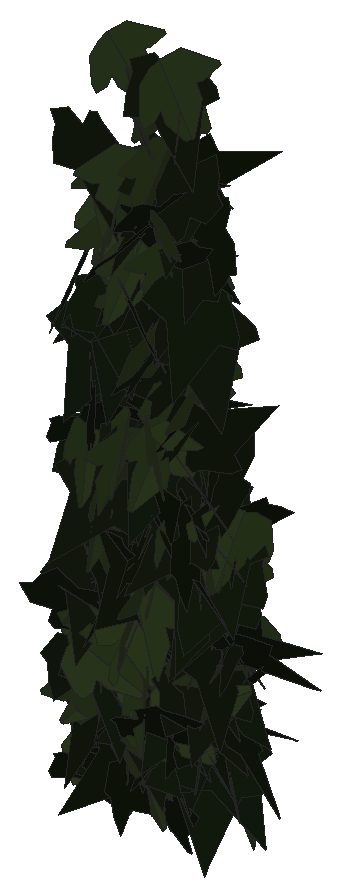
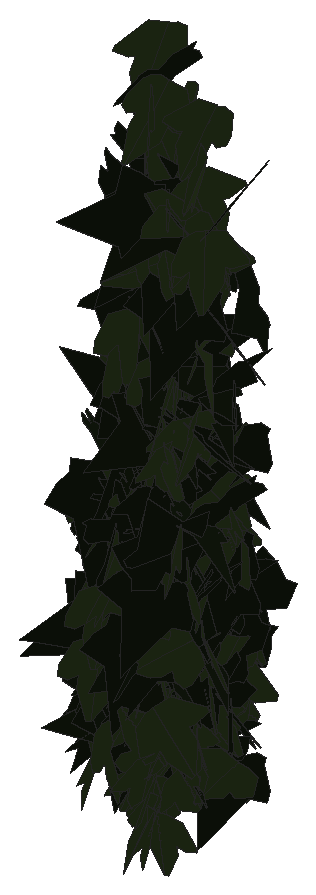
# SketchUp Ruby script. Lengths in inches.
U = 1.inch
M = Sketchup.active_model
def pt(a) = Geom::Point3d.new(a.map { |v| v * U })
def face(e, loops, mat)
  f = e.add_face(loops[0].map { |a| pt(a) })
  loops[1..].each { |l| e.add_face(l.map { |a| pt(a) }).erase! }
  f.material = f.back_material = mat if mat
  f
end
# faces: each face lists its corners as indices into pts; further lists are holes
def faces(e, pts, list, mat = nil) = list.each { |f| face(e, (f[0].is_a?(Array) ? f : [f]).map { |l| l.map { |i| pts[i] } }, mat) }
# xy, xz, yz: faces in a plane at the given z, y or x. An outline is a flat list of corners, or four numbers for a rectangle; further outlines are holes
def ring(l) = l.size == 4 ? [[l[0], l[1]], [l[2], l[1]], [l[2], l[3]], [l[0], l[3]]] : l.each_slice(2).to_a
def flat(e, list, mat, &to3) = list.each { |f| face(e, (f[0].is_a?(Array) ? f : [f]).map { |l| ring(l).map { |u, v| to3.(u, v) } }, mat) }
def xy(e, z, list, mat = nil) = flat(e, list, mat) { |x, y| [x, y, z] }
def xz(e, y, list, mat = nil) = flat(e, list, mat) { |x, z| [x, y, z] }
def yz(e, x, list, mat = nil) = flat(e, list, mat) { |y, z| [x, y, z] }
def lines(e, pts, list) = list.each { |a, b| e.add_line(pt(pts[a]), pt(pts[b])) }
# prism: a flat outline (further loops are holes) pulled along v
def prism(e, loops, v, mat = nil)
  f = face(e, loops, mat); d = Geom::Vector3d.new(v.map { |x| x * U })
  f.pushpull(f.normal.samedirection?(d) ? d.length : -d.length)
end
def box(e, o, s, mat = nil) = prism(e, [[o, [o[0] + s[0], o[1], o[2]], [o[0] + s[0], o[1] + s[1], o[2]], [o[0], o[1] + s[1], o[2]]]], [0, 0, s[2]], mat)
def at(x, y, z, deg = 0) = Geom::Transformation.translation(pt([x, y, z])) * Geom::Transformation.rotation(ORIGIN, Z_AXIS, deg.degrees)
def axes(o, x, y, z) = Geom::Transformation.new([*x, 0, *y, 0, *z, 0, *pt(o).to_a, 1])
def part(name) = M.definitions.add(name)
# library, detail: a bought-in or finely detailed component or shape, given as its bounding box
def library(name, o, s) = part(name).tap { |d| box(d.entities, o, s) }
def detail(e, o, s) = box(e.add_group.entities, o, s)
def put(e, d, t, mat = nil) = e.add_instance(d, t).tap { |i| i.material = mat if mat }
def group(e, t, mat = nil) = e.add_group.tap { |g| g.transformation = t; g.material = mat if mat }.entities
root = M.entities
M.materials.add("efeu1").color = [18, 25, 13]
M.materials.add("efeu2").color = [43, 57, 29]
c1 = part("ivyleaf_10")
p = [[0,0.5,-0.03],[-0.0625,2.02,-0.43],[-0.19,2.01,-0.46],[-0.54,1.05,-0.29],[-0.52,0.625,-0.18],[-0.83,0.76,-0.28],
  [-1.16,0.64,-0.33],[-1.15,0.33,-0.24],[-0.77,-0.39,0.02],[-0.3,-0.51,0.16],[0.04,-0.48,0.23],[-0.02,2.01,-0.4375],
  [-0.06,2.01,-0.43],[0.04,-0.49,0.23],[0.67,-0.49,0.14],[1.38,0.36,-0.2],[1.375,0.51,-0.24],[0.81,0.65,-0.19],
  [0.62,0.59,-0.15],[0.6,1.09,-0.28],[0.5,1.23,-0.31]]
faces(c1.entities,p,[[0,1,2,3,4,5,6,7,8,9,10],[11,12,0,13,14,15,16,17,18,19,20]],"efeu2")
c2 = part("ivyleaf_9")
p = [[1.54,2.16,1.25],[1.36,2.04,1.19],[-0.21,0.99,0.68],[-0.71,1.11,0.82],[-0.85,0.86,0.67],[-0.8,0.17,0.21],
  [-0.9,-0.01,0.1],[-0.67,-0.16,-0.02],[-0.08,-0.08,-0.05],[-0.03,-0.6,-0.4],[0.65,-0.88,-0.66],[0.83,-0.6,-0.49],
  [1.29,-0.42,-0.43],[1.8125,-0.07,-0.26],[1.21,0.44,0.15]]
faces(c2.entities,p,[[0,1,2,3,4,5,6,7,8,9,10,11,12,13,14]],"efeu1")
put(root,c1,axes([7.61,224.5,225.21],[0.35894,-0.31903,0.13922],[0.09481,-0.10282,-0.48004],[0.33492,0.37101,-0.01332]))
put(root,c1,axes([7.58,224.07,225.04],[0.18757,0.37221,0.14899],[0.06063,0.13188,-0.42714],[-0.42644,0.18247,0.00481]))
put(root,c1,axes([7.75,224.44,231.33],[-0.22715,-0.3782,-0.04595],[0.02733,0.03648,-0.45004],[0.41032,-0.2118,0.00454]))
put(root,c2,axes([7.99,224.41,227.15],[-0.21542,0.37118,0.11234],[-0.11464,0.06429,-0.4336],[-0.40145,-0.21753,0.06354]))
put(root,c1,axes([7.73,224.59,228.66],[0.07574,-0.26071,-0.35473],[0.02197,0.34723,-0.27168],[0.46313,0.02617,0.0709]))
put(root,c2,axes([7.83,223.22,229.9],[0.04008,0.18203,0.40907],[0.01412,0.39413,-0.19097],[-0.46787,0.02749,0.02928]))
put(root,c2,axes([7.56,224.16,223.65],[-0.02545,0.09105,0.4417],[0.06137,-0.42104,0.09715],[0.46508,0.06054,0.01135]))
put(root,c2,axes([7.57,224.38,227.42],[0.00542,-0.49083,-0.09518],[0.00382,0.09522,-0.49083],[0.49996,0.0046,0.00479]))
put(root,c1,axes([7.64,225.54,222.95],[0.46659,-0.00564,0.05248],[0.05452,0.0009,-0.44934],[0.00593,0.43496,0.00161]))
put(root,c1,axes([7.77,224.16,227.36],[0.17335,0.3156,-0.26281],[-0.12938,-0.22256,-0.3682],[-0.41704,0.20023,0.00498]))
put(root,c1,axes([7.8,225.07,227.125],[-0.37043,0.26625,0.02742],[-0.04567,-0.01161,-0.4501],[-0.28532,-0.34381,0.03644]))
put(root,c2,axes([7.73,223.81,223.13],[0.3453,0.28887,-0.06203],[-0.05186,-0.03581,-0.44809],[-0.31431,0.32326,0.00578]))
put(root,c1,axes([7.9,225.1875,224.25],[-0.17476,-0.34873,0.21168],[-0.08556,-0.18759,-0.39977],[0.42761,-0.18006,0.00652]))
put(root,c2,axes([8.05,224.07,225.14],[-0.1459,0.38314,0.16172],[-0.08247,0.13766,-0.42174],[-0.43889,-0.15324,0.02548]))
put(root,c2,axes([7.58,223.94,231.97],[0.19819,-0.45872,-0.01728],[-0.00253,0.01773,-0.49968],[0.45904,0.19815,0.0047]))
put(root,c1,axes([7.56,224.15,223.18],[0.3046,0.18868,0.28306],[0.23736,0.1608,-0.35278],[-0.26757,0.35745,0.00928]))
put(root,c1,axes([7.86,224.03,225.55],[-0.02783,-0.49665,-0.05061],[0.00726,0.05028,-0.49741],[0.49917,-0.02843,0.00442]))
put(root,c1,axes([7.76,224.79,228.71],[0.14203,0.41463,-0.00394],[-0.01303,-0.00014,-0.45223],[-0.44763,0.13156,0.01192]))
put(root,c1,axes([8.05,223.99,229.33],[-0.03318,0.19852,0.40127],[-0.34968,0.24702,-0.15899],[-0.31199,-0.29798,0.13553]))
put(root,c2,axes([7.84,224,226],[0.30337,0.30705,-0.13173],[-0.08637,-0.09848,-0.43273],[-0.34817,0.29197,-0.00743]))
put(root,c2,axes([7.82,224.1,224.2],[-0.40754,-0.06704,-0.28181],[0.28924,-0.0676,-0.40221],[0.01583,-0.49085,0.09388]))
put(root,c2,axes([7.74,223.61,224.93],[0.07038,-0.23683,-0.37337],[-0.11954,0.34165,-0.25528],[0.44885,0.12812,-0.00944]))
put(root,c2,axes([7.45,224,224.97],[0.22302,-0.1763,0.35345],[0.31425,-0.17869,-0.28028],[0.26874,0.35526,0.03443]))
put(root,c1,axes([7.85,223.74,226.28],[-0.43437,0.16544,-0.01004],[0.00865,-0.00591,-0.45228],[-0.17877,-0.40227,0.00252]))
put(root,c2,axes([7.78,224.18,229.08],[-0.14899,-0.43209,0.20273],[-0.02194,-0.20595,-0.45509],[0.47678,-0.1445,0.0424]))
put(root,c1,axes([8.01,224.08,224.32],[0.21632,0.21762,-0.33174],[-0.28496,-0.18523,-0.30374],[-0.30449,0.32796,0.04858]))
put(root,c1,axes([7.93,223.73,224.32],[-0.42115,-0.26938,-0.0083],[0.00407,0.00904,-0.4999],[0.26947,-0.42113,-0.00543]))
put(root,c2,axes([7.88,225.1,226.84],[-0.24224,-0.1765,0.3414],[0.27838,0.20327,0.29683],[-0.29075,0.34169,-0.00023]))
put(root,c1,axes([7.61,224.95,226.38],[0.22392,-0.13062,0.37379],[0.35999,-0.13865,-0.25238],[0.20242,0.39108,0.03536]))
put(root,c1,axes([7.82,224.49,232.58],[-0.27933,0.33329,-0.11032],[0.06892,-0.08475,-0.43874],[-0.3714,-0.26639,0.00156]))
put(root,c2,axes([8.1875,224.59,228.57],[-0.44129,0.12207,0.08927],[-0.10108,-0.01474,-0.44154],[-0.12552,-0.41726,0.04172]))
put(root,c1,axes([8.01,224.25,224.0625],[0.38812,0.09295,-0.23588],[-0.23564,-0.06213,-0.38601],[-0.12064,0.42039,-0.0049]))
put(root,c2,axes([7.92,223.91,225.8125],[0.12768,0.37309,0.19747],[0.06273,0.18078,-0.40703],[-0.44775,0.13171,-0.00071]))
put(root,c1,axes([7.85,225.43,222.92],[-0.16645,0.40487,-0.04095],[0.00816,-0.03925,-0.45049],[-0.43925,-0.15416,0.00715]))
put(root,c2,axes([7.85,223.58,228.125],[0.30554,0.33028,0.01032],[0.00708,0.00745,-0.45228],[-0.3568,0.28299,-0.00014]))
put(root,c1,axes([7.93,225.4375,223],[-0.13999,0.33376,0.25692],[-0.09144,0.23211,-0.37235],[-0.43904,-0.15476,-0.00437]))
put(root,c1,axes([8.04,224.125,224.58],[0.23939,-0.2391,-0.29948],[-0.17561,0.23993,-0.33735],[0.3641,0.27293,0.0342]))
put(root,c1,axes([7.9,224.76,223.25],[0.04747,0.37222,-0.22961],[-0.08439,-0.21144,-0.38692],[-0.45971,0.07725,0.04732]))
put(root,c1,axes([7.89,223.7,227.875],[0.07852,0.39784,-0.16661],[-0.02727,-0.15823,-0.42059],[-0.46239,0.07689,-0.00349]))
put(root,c1,axes([7.8,225.01,227.94],[0.22296,-0.35751,-0.14257],[0.07711,-0.11706,0.42934],[-0.40627,-0.21842,0.00325]))
put(root,c2,axes([7.5625,223.43,225.39],[0.14224,-0.0871,0.42154],[0.44001,-0.05156,-0.1492],[0.08291,0.42306,0.0686]))
put(root,c2,axes([8.21,224.7,228.48],[-0.44022,-0.05088,0.14886],[-0.14545,-0.06858,-0.42422],[0.0759,-0.42654,0.05045]))
put(root,c2,axes([7.93,223.71,226.42],[0.39807,0.13767,-0.19294],[-0.19397,-0.04895,-0.40888],[-0.15693,0.40973,0.01597]))
put(root,c1,axes([7.86,225.42,223.04],[-0.22501,0.34827,-0.16287],[0.08093,-0.13764,-0.42202],[-0.40439,-0.22133,0.00617]))
put(root,c2,axes([7.85,225.18,226.67],[0.30659,0.24189,0.23285],[-0.20101,-0.12623,0.38725],[0.29379,-0.3388,0.02196]))
put(root,c2,axes([7.73,224.65,228.18],[0.15735,-0.4086,0.03366],[0.01971,-0.02785,-0.45107],[0.44223,0.14662,0.00813]))
put(root,c2,axes([7.89,223.875,225.9],[-0.13806,-0.41381,0.04223],[-0.01431,-0.0384,-0.45042],[0.44883,-0.12851,-0.00137]))
put(root,c2,axes([7.65,224.32,224.29],[-0.01325,-0.0949,0.44132],[0.46657,-0.05094,0.00114],[0.05341,0.42146,0.09951]))
put(root,c1,axes([8.05,223.89,226.66],[-0.33491,-0.30505,-0.00273],[-0.0001,0.00383,-0.45238],[0.32946,-0.31009,-0.00291]))
put(root,c1,axes([7.96,225.38,223.27],[-0.21708,0.38487,-0.02748],[-0.00924,-0.03423,-0.45091],[-0.41654,-0.19982,0.02433]))
put(root,c1,axes([7.92,224.16,233.16],[0.17949,0.3432,0.2177],[-0.00285,0.22743,-0.38563],[-0.43415,0.1404,0.09254]))
put(root,c1,axes([8.17,223.5,225.22],[0.36409,-0.04043,-0.2828],[-0.28527,0.07166,-0.35164],[0.08232,0.42715,0.03222]))
put(root,c2,axes([8.21,223.84,229.11],[-0.19624,0.45873,0.03253],[-0.00754,0.03216,-0.49891],[-0.45982,-0.1963,-0.0057]))
put(root,c1,axes([7.69,225.04,225.4375],[0.28719,0.00254,0.35802],[0.31618,0.22719,-0.23694],[-0.19561,0.37095,0.14266]))
put(root,c1,axes([7.94,224.11,224.57],[0.1516,0.40842,-0.05418],[-0.02607,-0.04678,-0.44907],[-0.4439,0.14223,0.00787]))
put(root,c2,axes([8.24,223.94,230.13],[-0.46658,0.17785,-0.02602],[0.02806,0.00058,-0.49921],[-0.17754,-0.4673,-0.01052]))
put(root,c1,axes([7.93,223.85,227.09],[0.38214,-0.23782,0.08986],[0.07415,-0.05274,-0.44335],[0.26303,0.36039,-0.00558]))
put(root,c1,axes([7.96,224.91,228.34],[0.06858,0.42066,-0.09441],[-0.01439,-0.0898,-0.44244],[-0.46454,0.06488,-0.00023]))
put(root,c2,axes([7.97,225.16,226.3],[0.36574,0.2637,-0.07356],[-0.05036,-0.05517,-0.44612],[-0.29053,0.34153,-0.01526]))
put(root,c1,axes([8.12,224.53,223.6875],[-0.2118,-0.43639,0.12128],[-0.03301,-0.11865,-0.48459],[0.45172,-0.21328,0.02145]))
put(root,c1,axes([8,225.35,223.64],[0.03854,0.43344,0.00927],[0.00167,0.00882,-0.4523],[-0.46821,0.03571,-0.00085]))
put(root,c2,axes([8.22,223.27,228.19],[0.04121,-0.07593,0.44368],[-0.05238,0.42483,0.08315],[-0.46505,-0.05458,0.02996]))
put(root,c1,axes([8.01,225.23,223.76],[-0.0485,-0.38273,0.20987],[0.01715,0.20129,0.40071],[-0.46697,0.04715,-0.00709]))
put(root,c2,axes([7.73,224.21,225.26],[0.31805,-0.34067,0.18108],[0.15967,-0.09741,-0.4637],[0.35121,0.35279,0.04683]))
put(root,c2,axes([8.03,223.9,225.5625],[0.19457,0.27668,0.29455],[0.12601,0.26025,-0.34159],[-0.40863,0.212,0.03492]))
put(root,c1,axes([8.18,223.94,230.83],[-0.22175,-0.44636,0.03986],[-0.004,-0.0425,-0.49817],[0.44812,-0.22126,0.01528]))
put(root,c1,axes([8.07,223.77,226.95],[-0.03273,0.33799,-0.28304],[-0.0189,-0.27355,-0.35128],[-0.46828,-0.01259,0.03396]))
put(root,c2,axes([8.32,224.58,228.92],[-0.19055,0.39684,-0.02578],[0.00811,-0.02379,-0.45166],[-0.42935,-0.17657,0.00291]))
put(root,c2,axes([8.16,224.49,228.77],[-0.40195,-0.20988,-0.0849],[0.11545,-0.02585,-0.4377],[0.21406,-0.38014,0.07664]))
put(root,c1,axes([8.11,223.79,231.11],[0.32841,-0.30981,0.02892],[0.02321,-0.01787,-0.45147],[0.33514,0.30483,0.00293]))
put(root,c2,axes([7.99,224.07,224.72],[-0.03115,-0.49476,-0.06516],[0.00966,0.06468,-0.4957],[0.49894,-0.03214,0.00553]))
put(root,c1,axes([8.14,224.67,228.99],[0.1108,-0.27768,-0.33149],[0.03153,0.33186,-0.29091],[0.45546,0.04458,0.10078]))
put(root,c2,axes([8.12,224.04,223.09],[-0.3553,-0.06116,0.28907],[0.30072,0.01872,0.34703],[-0.06359,0.43027,0.02599]))
put(root,c2,axes([8.29,223.64,227.35],[-0.45345,-0.10979,-0.031],[0.03049,0.00987,-0.45133],[0.11902,-0.4208,-0.0025]))
put(root,c2,axes([8.03,223.97,225.94],[0.24739,-0.28343,-0.24704],[-0.16121,0.18478,-0.379],[0.36541,0.27341,0.00005]))
put(root,c1,axes([8.11,224.31,223.5625],[0.02926,-0.34085,0.27966],[0.11039,-0.25685,-0.3493],[0.45571,0.0841,0.06666]))
put(root,c2,axes([8.06,224.18,229.4375],[-0.09459,-0.49001,0.03076],[-0.01006,-0.02939,-0.49903],[0.49087,-0.09502,-0.0043]))
put(root,c2,axes([7.98,224.51,225.68],[0.09626,-0.49064,0.00219],[0.00039,-0.00215,-0.5],[0.49065,0.09627,-0.00003]))
put(root,c1,axes([8.2,224.625,228.96],[-0.33818,0.30184,-0.00856],[-0.04218,-0.05224,-0.44729],[-0.32337,-0.30885,0.06729]))
put(root,c2,axes([8.23,224.44,224.59],[-0.35091,0.07466,-0.2906],[0.25343,-0.17763,-0.33314],[-0.18261,-0.39,0.0961]))
put(root,c1,axes([8.24,224.2,224.51],[0.05162,-0.41708,0.11852],[0.03448,-0.11094,-0.43618],[0.46568,0.05445,0.01916]))
put(root,c1,axes([8.28,224.91,225.8],[-0.42284,0.18372,0.04866],[-0.05446,0.00257,-0.44934],[-0.19737,-0.39429,0.01974]))
put(root,c1,axes([8.27,224.26,231.46],[-0.43676,-0.15527,-0.0412],[0.03889,0.01674,-0.45051],[0.16863,-0.406,-0.00281]))
put(root,c2,axes([8.41,224.4,224.35],[-0.06273,0.42947,-0.03898],[-0.00471,-0.03841,-0.45061],[-0.46557,-0.05748,0.00982]))
put(root,c1,axes([8.18,223.88,231.0625],[0.45737,0.09911,0.00776],[0.00729,0.00389,-0.45233],[-0.1071,0.42354,0.00234]))
put(root,c1,axes([8.4,224.16,223.85],[-0.42839,-0.14086,0.11413],[-0.10976,-0.04171,-0.43774],[0.15857,-0.40944,0.00533]))
put(root,c2,axes([8.13,224.4375,226.36],[-0.04349,-0.49765,-0.02135],[0.00335,0.02113,-0.49954],[0.49809,-0.04359,0.00149]))
put(root,c2,axes([8.13,223.95,229.83],[-0.16099,-0.36088,-0.19943],[0.12995,0.15632,-0.40321],[0.42179,-0.1859,0.0481]))
put(root,c1,axes([8.03,224.2,223.5625],[0.11829,-0.10108,0.42502],[0.34507,-0.255,-0.15466],[0.29605,0.33762,0.01044]))
put(root,c1,axes([8.34,223.92,231.74],[-0.20476,-0.41564,0.18793],[0.00294,-0.2072,-0.45504],[0.45614,-0.18524,0.08729]))
put(root,c1,axes([8.29,224.03,229.15],[-0.25571,0.36272,0.04159],[-0.0315,0.0287,-0.45039],[-0.39285,-0.2384,0.00905]))
put(root,c2,axes([8.28,224.11,230.23],[0.37524,0.31312,-0.10559],[-0.11729,-0.02316,-0.4855],[-0.30892,0.38913,0.05607]))
put(root,c1,axes([8.36,224.25,230.9],[-0.06658,-0.3968,0.17395],[-0.01242,-0.16738,-0.4174],[0.46489,-0.0613,0.01376]))
put(root,c2,axes([8.51,224.25,227.93],[-0.49837,0.01119,-0.03877],[0.03888,0.00457,-0.49847],[-0.0108,-0.49985,-0.00542]))
put(root,c2,axes([7.97,223.86,222.93],[0.34235,0.04231,0.30667],[0.31579,0.03815,-0.33259],[-0.06153,0.43125,-0.00067]))
put(root,c2,axes([8.38,224.74,227.11],[-0.40489,-0.16209,-0.15567],[0.14835,0.05948,-0.42477],[0.18647,-0.39927,-0.00008]))
put(root,c2,axes([8.33,225.11,225.3],[0.34371,0.27644,-0.11164],[-0.0781,-0.08036,-0.43821],[-0.3106,0.32611,-0.01335]))
put(root,c1,axes([8.42,224.42,222.97],[-0.4695,-0.01324,0.00854],[-0.0088,-0.00222,-0.45231],[0.01434,-0.43479,0.00205]))
put(root,c2,axes([8.23,224.84,227.56],[-0.05882,-0.38552,-0.20176],[0.03162,0.19178,-0.40492],[0.46503,-0.06181,0.00201]))
put(root,c2,axes([8.4,223.85,223.45],[-0.02052,-0.09245,-0.44162],[0.17712,-0.39514,0.08183],[-0.43465,-0.15665,0.05419]))
put(root,c2,axes([8.49,223.52,230.75],[0.10655,0.45238,0.18439],[-0.02433,0.1934,-0.46044],[-0.48791,0.08915,0.06322]))
put(root,c1,axes([8.35,225.0625,225.64],[-0.14164,0.41358,-0.03248],[0.002,-0.03217,-0.45116],[-0.44793,-0.13092,0.00826]))
put(root,c1,axes([8.33,223.89,229.78],[-0.38255,-0.19027,-0.17263],[0.17746,0.04342,-0.41644],[0.20705,-0.38876,0.03798]))
put(root,c1,axes([8.24,224.25,223.1],[-0.30777,0.11338,-0.32082],[0.24081,-0.23326,-0.30338],[-0.26076,-0.34923,0.09848]))
put(root,c1,axes([8.49,223.76,227.9],[-0.05191,-0.45652,0.19721],[-0.01809,-0.19642,-0.45945],[0.49697,-0.05484,0.00388]))
put(root,c1,axes([8.2,223.27,225.06],[0.21413,0.19013,0.35078],[0.2136,0.27604,-0.28274],[-0.35949,0.27727,0.04094]))
put(root,c2,axes([8.48,223.57,223.46],[0.19308,-0.1422,-0.43875],[-0.33484,0.28388,-0.23936],[0.31718,0.38625,0.0144]))
put(root,c1,axes([8.48,224.52,224.96],[0.19428,-0.45763,-0.05317],[-0.0131,0.05219,-0.4971],[0.46053,0.19455,0.00829]))
put(root,c2,axes([8.74,224.06,223.61],[-0.26681,0.40998,0.10357],[-0.06647,0.08028,-0.48902],[-0.4176,-0.27472,0.01167]))
put(root,c1,axes([8.5,223.84,230.52],[0.19886,0.33603,-0.21416],[-0.14134,-0.16226,-0.39707],[-0.40148,0.22356,0.03371]))
put(root,c1,axes([8.375,225.04,223.875],[-0.3747,0.20373,-0.172],[0.13956,-0.10596,-0.41768],[-0.24665,-0.36945,0.02495]))
put(root,c1,axes([8.52,224.31,227.79],[0.02447,-0.4637,-0.18544],[0.01344,0.18621,-0.46384],[0.49922,0.01772,0.02158]))
put(root,c2,axes([8.14,224.25,224.91],[0.40084,-0.16238,0.1648],[0.15737,-0.06228,-0.42131],[0.18782,0.39872,0.00131]))
put(root,c1,axes([8.54,224.66,223.29],[-0.05366,-0.48467,0.11052],[0.00168,-0.11134,-0.48744],[0.49711,-0.05194,0.01357]))
put(root,c1,axes([8.3,224.07,225.63],[-0.05451,-0.13591,-0.42653],[0.31958,0.29001,-0.13782],[0.34002,-0.29436,0.06116]))
put(root,c2,axes([8.71,224.59,223.82],[-0.14377,0.3668,-0.30788],[-0.01127,-0.32395,-0.38069],[-0.47875,-0.10253,0.10141]))
put(root,c1,axes([8.71,224.37,231.56],[-0.37469,-0.1029,0.25105],[-0.1938,-0.19895,-0.35641],[0.20679,-0.3729,0.12087]))
put(root,c2,axes([8.57,223.83,226.48],[-0.36875,0.12368,-0.3142],[0.26057,-0.19169,-0.38126],[-0.21477,-0.44493,0.07692]))
put(root,c1,axes([8.43,224.02,224.55],[-0.3925,0.20013,-0.13597],[0.12734,-0.0569,-0.43143],[-0.22459,-0.38202,-0.00698]))
put(root,c2,axes([8.73,224.05,226.67],[-0.27793,0.33672,-0.10198],[0.02647,-0.10406,-0.43852],[-0.37784,-0.25498,0.04429]))
put(root,c1,axes([8.61,223.92,226.13],[0.30663,-0.27257,-0.19267],[-0.12998,0.14189,-0.40893],[0.33135,0.30789,0.01789]))
put(root,c1,axes([8.45,225.06,225.91],[0.44671,-0.12498,0.05221],[0.05074,-0.01808,-0.44936],[0.13633,0.41627,-0.00384]))
put(root,c2,axes([8.43,223.92,225.96],[-0.04056,-0.29488,0.40175],[-0.04473,-0.3993,-0.29759],[0.49634,-0.06008,0.00601]))
put(root,c1,axes([8.48,224.34,225.32],[0.19372,0.39406,-0.04374],[-0.02728,-0.0347,-0.45019],[-0.42713,0.18094,0.00892]))
put(root,c1,axes([8.45,223.61,228.19],[0.32291,-0.28501,0.14182],[0.115,-0.08587,-0.42945],[0.32127,0.3172,0.01118]))
put(root,c1,axes([8.6,224.6,224.84],[-0.30012,0.31034,0.13028],[-0.09019,0.09337,-0.43324],[-0.35001,-0.29017,-0.00007]))
put(root,c2,axes([8.54,223.99,231.09],[0.36618,0.32291,-0.10791],[-0.08911,-0.06206,-0.48807],[-0.3286,0.37667,0.0121]))
put(root,c2,axes([8.6,224.14,231.5],[-0.38664,-0.02733,-0.25541],[0.26229,-0.11871,-0.35444],[-0.04925,-0.4176,0.11748]))
put(root,c2,axes([8.74,224.15,226.06],[-0.02055,0.42918,0.07108],[-0.01462,0.06779,-0.44665],[-0.46912,-0.02091,0.01081]))
put(root,c2,axes([8.52,224.54,226.75],[-0.26161,-0.36102,-0.01502],[0.12804,-0.06299,-0.43032],[0.36861,-0.23435,0.13881]))
put(root,c1,axes([8.57,224.57,223.39],[0.35801,0.32689,-0.12236],[-0.08071,-0.093,-0.4846],[-0.33958,0.36673,-0.01382]))
put(root,c1,axes([8.71,223.77,227.84],[0.07057,-0.27685,-0.34227],[-0.085,0.31956,-0.29583],[0.45662,0.10228,-0.00217]))
put(root,c2,axes([8.49,224.03,224.06],[-0.05661,-0.40052,-0.16789],[0.02155,0.1602,-0.42009],[0.46588,-0.05608,-0.00097]))
put(root,c1,axes([8.68,224.59,225.83],[-0.06885,-0.40709,0.14501],[-0.00608,-0.14015,-0.42824],[0.46469,-0.06215,0.01588]))
put(root,c1,axes([8.7,224.17,228.93],[-0.21751,-0.44316,-0.07935],[0.02266,0.07723,-0.49348],[0.44964,-0.21827,-0.01351]))
put(root,c1,axes([8.64,223.84,225.79],[0.16384,-0.43539,0.18329],[0.05552,-0.17491,-0.46511],[0.46912,0.17276,-0.00897]))
put(root,c1,axes([8.57,224.65,223.46],[0.22737,0.39632,0.20306],[0.00815,0.22426,-0.44681],[-0.44524,0.20649,0.09552]))
put(root,c1,axes([8.72,224.57,223.87],[-0.03246,-0.43508,0.24425],[0.01425,-0.24547,-0.43536],[0.49874,-0.02131,0.02833]))
put(root,c2,axes([8.62,224.29,227.72],[-0.1338,-0.46252,0.13481],[-0.03032,-0.13155,-0.48143],[0.48081,-0.137,0.00715]))
put(root,c1,axes([8.51,224.23,227],[0.43429,-0.02337,0.17082],[0.17782,0.0032,-0.41873],[0.02206,0.43436,0.01227]))
put(root,c1,axes([8.64,224.34,224.83],[0.18838,0.3926,-0.07102],[-0.03283,-0.06122,-0.44678],[-0.42912,0.17704,0.00301]))
put(root,c1,axes([8.75,225.17,223.72],[-0.0756,-0.42916,-0.01245],[0.00545,0.0113,-0.45222],[0.46364,-0.07011,0.00328]))
put(root,c1,axes([8.75,224.43,231.08],[-0.27443,-0.34579,0.0742],[0.0175,-0.09922,-0.44015],[0.38091,-0.24456,0.07367]))
put(root,c2,axes([8.96,223.83,230.23],[-0.40297,0.2193,-0.04552],[-0.00147,-0.08736,-0.44318],[-0.24151,-0.36538,0.07864]))
put(root,c1,axes([8.65,224.65,223.15],[-0.00788,0.49993,-0.00313],[0.00402,-0.00307,-0.49997],[-0.49992,-0.00791,-0.00397]))
put(root,c2,axes([8.56,224.33,228.21],[0.34862,0.19408,0.22633],[0.1273,0.2101,-0.37669],[-0.28805,0.32774,0.10745]))
put(root,c1,axes([8.7,224.59,223.91],[-0.10719,0.48836,-0.00419],[0.00352,-0.00352,-0.49998],[-0.48836,-0.10721,-0.00268]))
put(root,c1,axes([8.71,224.59,223.89],[0.15031,-0.40025,0.25924],[0.09068,-0.24286,-0.42755],[0.46817,0.17555,-0.00042]))
put(root,c1,axes([8.63,223.72,223.64],[-0.4068,-0.13907,-0.2553],[0.23721,0.09506,-0.42976],[0.16807,-0.47077,-0.01137]))
put(root,c2,axes([8.48,225.17,225.07],[0.38894,-0.24121,0.03819],[0.0263,-0.0296,-0.45064],[0.26219,0.36079,-0.01145]))
put(root,c1,axes([8.8,223.45,232.83],[-0.30929,0.30647,0.11988],[-0.07395,0.0937,-0.436],[-0.34581,-0.29414,-0.01399]))
put(root,c2,axes([8.65,224.2,231.49],[0.39801,0.22646,0.04795],[-0.01516,0.10856,-0.43784],[-0.24913,0.35519,0.10325]))
put(root,c1,axes([8.54,224.01,224.36],[0.28009,0.21913,0.28282],[0.21637,0.1841,-0.35298],[-0.30895,0.32759,0.00919]))
put(root,c1,axes([8.69,224.39,229.76],[0.31363,-0.28753,0.15504],[0.12659,-0.09335,-0.42471],[0.32608,0.31279,0.01576]))
put(root,c2,axes([8.86,224.57,223.89],[0.20062,0.45392,-0.06094],[-0.01984,-0.05786,-0.49625],[-0.45756,0.20153,-0.0052]))
put(root,c1,axes([8.87,224.53,224.41],[-0.3985,0.29823,0.04745],[-0.03925,0.02674,-0.49774],[-0.29942,-0.40043,0.0021]))
put(root,c2,axes([9.01,224.11,228.4375],[0.22633,0.27301,-0.35248],[-0.27172,-0.22893,-0.35179],[-0.35347,0.35079,0.04473]))
put(root,c2,axes([8.91,224.97,226.93],[-0.32674,-0.31093,0.03323],[-0.03154,-0.01615,-0.45107],[0.33609,-0.30379,-0.01003]))
put(root,c1,axes([8.61,223.74,224.66],[0.30647,-0.19149,0.34556],[0.30006,-0.17167,-0.36124],[0.25699,0.42879,0.00969]))
put(root,c2,axes([8.8,223.36,230.14],[0.37161,-0.10309,-0.25518],[-0.25249,0.07457,-0.37354],[0.13736,0.41598,0.00372]))
put(root,c1,axes([8.69,223.58,225.72],[0.4319,0.19404,0.16066],[0.1354,0.0901,-0.47281],[-0.21244,0.45192,0.02528]))
put(root,c2,axes([9.09,223.44,229.6],[-0.30087,0.33219,-0.03699],[0.03026,-0.02291,-0.45083],[-0.35955,-0.27991,-0.007]))
put(root,c2,axes([9.09,223.63,228.84],[-0.13688,0.41187,0.06173],[-0.03094,0.05326,-0.44801],[-0.44835,-0.12942,0.01207]))
put(root,c2,axes([9.06,224.46,225.16],[-0.20091,-0.41728,0.18844],[0.07622,0.17243,0.4631],[-0.45147,0.21481,-0.00568]))
put(root,c2,axes([9.11,224.42,223.41],[-0.26486,0.33196,-0.14291],[0.00934,-0.16087,-0.42023],[-0.38791,-0.23053,0.08746]))
put(root,c2,axes([8.61,224.26,222.58],[0.03522,-0.08486,0.44241],[0.23361,-0.36659,-0.0933],[0.40607,0.21826,0.01531]))
put(root,c2,axes([8.875,224.53,224.29],[-0.2353,-0.40967,0.16372],[0.00489,-0.18797,-0.4633],[0.44115,-0.21643,0.09246]))
put(root,c1,axes([8.94,223.79,232.17],[-0.00746,-0.47089,0.16795],[0.0273,-0.1681,-0.4701],[0.4992,0.00215,0.02822]))
put(root,c1,axes([8.93,223.78,228.06],[0.15402,0.33324,-0.25012],[-0.10807,-0.21875,-0.37693],[-0.43048,0.17414,0.00514]))
put(root,c1,axes([8.98,224.51,224.53],[-0.0174,-0.49436,-0.07287],[-0.01223,0.07331,-0.49444],[0.49955,-0.01543,-0.01464]))
put(root,c1,axes([8.88,224.51,224.5625],[-0.18483,0.46249,-0.04407],[0.01216,-0.0426,-0.49803],[-0.46442,-0.18517,0.0045]))
put(root,c1,axes([8.97,225.11,225.6875],[-0.31167,-0.32014,-0.0611],[0.05212,0.03557,-0.44808],[0.34764,-0.29235,0.0124]))
put(root,c2,axes([8.73,224.56,224],[0.14371,-0.10725,-0.46674],[0.37675,-0.27551,0.17931],[-0.29565,-0.40323,0.00162]))
put(root,c1,axes([8.92,223.68,228.32],[-0.11871,0.41778,-0.05303],[0.00364,-0.05182,-0.44916],[-0.45454,-0.10952,0.01025]))
put(root,c1,axes([9.01,223.41,229.67],[-0.05773,-0.36198,-0.24465],[0.02125,0.23475,-0.38032],[0.46575,-0.05558,-0.01298]))
put(root,c1,axes([8.92,225.05,225.97],[-0.1367,0.41243,-0.05796],[0.0282,-0.05027,-0.44855],[-0.44859,-0.12884,-0.01053]))
put(root,c2,axes([8.76,224.4375,231.44],[0.16768,0.11303,0.40592],[0.35228,0.21451,-0.19955],[-0.26171,0.36116,-0.00852]))
put(root,c1,axes([9.03,223.56,231.35],[-0.38708,0.24196,0.04902],[-0.04196,0.02669,-0.44974],[-0.2629,-0.36051,-0.00039]))
put(root,c2,axes([9.18,224.06,228.375],[-0.37012,0.2309,-0.1413],[0.08525,-0.12378,-0.42586],[-0.2765,-0.34726,0.05784]))
put(root,c1,axes([8.85,224.23,224.7],[0.16731,-0.29447,0.29141],[0.23355,-0.1942,-0.33659],[0.37172,0.25455,0.08032]))
put(root,c1,axes([9.06,225.12,224.86],[-0.36925,-0.26632,-0.03898],[0.03337,0.02132,-0.45071],[0.28854,-0.34328,0.00225]))
put(root,c2,axes([9.1,223.58,231.54],[0.14304,0.39668,-0.12449],[-0.03832,-0.11435,-0.43493],[-0.44585,0.13709,-0.00256]))
put(root,c2,axes([8.95,224.18,231.7],[-0.22219,-0.37564,-0.07915],[0.07244,0.04976,-0.44398],[0.40755,-0.21364,0.03577]))
put(root,c2,axes([8.65,224.6,223.85],[0.42366,-0.09197,0.24911],[0.26446,0.1038,-0.41144],[0.02397,0.48038,0.1366]))
put(root,c2,axes([8.79,223.85,226.95],[-0.04135,0.01254,0.45046],[0.19167,-0.39622,0.02825],[0.42692,0.1791,0.03095]))
put(root,c2,axes([8.91,224.49,224.08],[-0.05353,-0.49664,-0.02201],[-0.00127,0.02227,-0.4995],[0.49713,-0.05342,-0.00365]))
put(root,c2,axes([9.18,224.375,223.89],[0.07577,0.42873,-0.02317],[-0.07575,-0.01082,-0.44634],[-0.45742,0.07281,0.07008]))
put(root,c1,axes([9,223.83,232.97],[-0.19216,-0.34355,-0.3083],[0.1337,0.27821,-0.39335],[0.44181,-0.23361,-0.01506]))
put(root,c1,axes([9.125,223.79,230.8125],[-0.15265,-0.39922,0.10332],[-0.03708,-0.09323,-0.44044],[0.44276,-0.14545,-0.00127]))
put(root,c2,axes([9.13,224.07,228.625],[0.31071,0.21773,-0.25272],[-0.25687,-0.08183,-0.3691],[-0.24122,0.36759,0.06753]))
put(root,c1,axes([9.1,224.48,223.57],[-0.35456,0.2822,0.04423],[-0.06,0.00039,-0.44869],[-0.30232,-0.33104,0.03718]))
put(root,c2,axes([9.4,223.62,229.375],[-0.35876,0.30973,0.15925],[-0.14218,0.07845,-0.47289],[-0.31793,-0.38459,0.03179]))
put(root,c2,axes([8.79,224.56,224.19],[0.25102,-0.42312,0.08921],[0.04751,-0.07554,-0.49197],[0.4298,0.25547,0.00228]))
put(root,c2,axes([8.9,223.45,224.24],[0.41762,0.1881,0.06836],[0.05686,0.04195,-0.44695],[-0.20755,0.38998,0.01511]))
put(root,c1,axes([8.74,224.39,230.69],[0.24352,0.00965,0.38675],[0.38461,0.12011,-0.2278],[-0.11614,0.41798,0.05654]))
put(root,c2,axes([9.22,223.98,228.37],[-0.01858,0.43288,0.04089],[0.00405,0.0395,-0.45051],[-0.46942,-0.01679,-0.0055]))
put(root,c1,axes([8.86,224.92,226.39],[0.32097,-0.21271,0.24535],[0.27986,-0.0245,-0.36248],[0.19842,0.37865,0.11437]))
put(root,c2,axes([8.92,224.32,223.91],[0.25724,-0.31993,-0.18055],[-0.0941,0.15133,-0.41435],[0.38169,0.25292,0.01953]))
put(root,c1,axes([9.13,224.46,226.42],[-0.45549,0.10653,-0.00116],[0.0012,-0.00018,-0.4524],[-0.11506,-0.42175,-0.0001]))
put(root,c1,axes([9.14,224.48,225.1],[0.16651,-0.44273,-0.16207],[-0.00544,0.17006,-0.47016],[0.47143,0.15834,0.05182]))
put(root,c2,axes([9.51,224.29,226.66],[-0.2281,0.00704,-0.44488],[-0.43393,-0.11405,0.22068],[-0.09837,0.48677,0.05814]))
put(root,c1,axes([9.11,223.9375,226.88],[0.12301,0.39761,0.14015],[-0.09277,0.15875,-0.41162],[-0.44382,0.07702,0.12488]))
put(root,c2,axes([9.3125,223.98,227.03],[-0.45869,-0.09293,-0.01484],[0.02094,-0.02194,-0.45137],[0.09936,-0.42439,0.02659]))
put(root,c2,axes([8.93,224.52,224.68],[0.00365,-0.27395,-0.41826],[0.137,0.40281,-0.26263],[0.48085,-0.11268,0.078]))
put(root,c1,axes([9.2,224.17,226.61],[0.05082,-0.42651,-0.07425],[0.00588,0.0724,-0.44605],[0.46701,0.0455,0.0137]))
put(root,c1,axes([9.18,223.85,232.9],[0.27813,-0.36944,-0.19015],[-0.00639,0.22499,-0.44647],[0.41546,0.25078,0.12043]))
put(root,c2,axes([9.4375,224.43,225.01],[-0.17643,0.37098,0.16414],[-0.06032,0.14782,-0.42149],[-0.43121,-0.17247,-0.00819]))
put(root,c2,axes([8.93,224.01,226.68],[0.32036,-0.31469,0.04885],[0.03343,-0.03538,-0.44975],[0.342,0.29823,-0.0018]))
put(root,c1,axes([9.3,224.55,223.71],[-0.06148,-0.48825,0.08849],[-0.02259,-0.08632,-0.49197],[0.49569,-0.06449,-0.01145]))
put(root,c1,axes([9.3,223.97,229.34],[-0.44295,-0.23144,0.01509],[-0.01159,-0.01039,-0.49976],[0.23164,-0.44309,0.00384]))
put(root,c2,axes([9.4375,224.48,225.07],[-0.43682,0.14937,-0.05995],[0.05379,-0.03147,-0.44823],[-0.16434,-0.40734,0.01264]))
put(root,c1,axes([9.3,224.28,226.36],[-0.40156,-0.22569,-0.0068],[0.00577,0.0038,-0.45235],[0.24378,-0.37185,-0.0005]))
put(root,c2,axes([9.36,224.38,225.94],[-0.06051,-0.30317,0.39297],[0.08217,0.38429,0.30914],[-0.48948,0.102,0.00331]))
put(root,c2,axes([9.54,223.57,231.64],[0.0246,0.15811,0.42079],[-0.32574,0.29734,-0.10319],[-0.33764,-0.27534,0.1302]))
put(root,c2,axes([9.08,223.78,233.34],[0.05922,-0.48083,-0.12369],[-0.01201,0.12315,-0.48445],[0.49634,0.06035,0.00303]))
put(root,c2,axes([9.27,223.98,230.77],[-0.43348,-0.10269,-0.22704],[0.22642,0.02794,-0.44492],[0.10406,-0.48854,0.02228]))
put(root,c2,axes([9.43,224.56,224.3],[-0.039,0.43092,0.04909],[-0.01228,0.0464,-0.44966],[-0.46802,-0.03713,0.00771]))
put(root,c2,axes([9.15,223.73,230.76],[0.37266,0.25743,0.06489],[0.06176,0.02765,-0.44755],[-0.27933,0.34956,-0.01239]))
put(root,c1,axes([9.35,224.29,225.5625],[-0.37451,-0.26237,-0.0123],[0.00996,0.00742,-0.45223],[0.28347,-0.34689,-0.00037]))
put(root,c1,axes([9.39,224.32,224.61],[-0.17219,-0.44366,0.15336],[-0.03659,-0.15016,-0.47551],[0.46799,-0.17498,0.01925]))
put(root,c1,axes([9.11,223.66,228.46],[-0.13421,-0.17882,0.39163],[0.20858,0.32353,0.22607],[-0.39899,0.22929,-0.01356]))
put(root,c1,axes([9.18,224.33,223.97],[0.28346,-0.27464,0.22041],[0.16968,-0.14283,-0.39485],[0.33403,0.30561,0.01354]))
put(root,c2,axes([9.15,224.1,224.69],[0.18339,-0.38326,-0.26359],[-0.05776,0.26238,-0.42169],[0.46155,0.18512,0.05196]))
put(root,c1,axes([9.4,224.1,228.82],[-0.03345,-0.48428,-0.1198],[-0.00572,0.12043,-0.48525],[0.49885,-0.0311,-0.0136]))
put(root,c2,axes([9.26,224.37,223.4375],[-0.16041,-0.4594,-0.11499],[0.04513,0.10603,-0.48654],[0.47141,-0.16647,0.00745]))
put(root,c2,axes([9.1,224.27,227],[0.36521,-0.27326,-0.01493],[-0.00442,0.01778,-0.452],[0.29549,0.33799,0.0117]))
put(root,c2,axes([9.43,223.57,226.97],[0.17987,-0.06917,-0.46137],[-0.37643,0.27057,-0.18732],[0.27558,0.41474,0.04526]))
put(root,c1,axes([9.05,223.92,224.125],[0.23927,-0.02431,-0.43836],[0.41767,0.16646,0.21874],[0.1353,-0.47085,0.09996]))
put(root,c1,axes([9.4,224.34,224.66],[0.16968,-0.44357,-0.15639],[0.04452,0.18066,-0.46409],[0.46822,0.14357,0.1008]))
put(root,c2,axes([9.52,224.34,226.61],[-0.08411,-0.32447,0.37101],[0.09187,0.35946,0.33519],[-0.48424,0.12455,-0.00086]))
put(root,c2,axes([9.34,224.2,226.01],[-0.10811,-0.40107,0.14088],[-0.03845,-0.13073,-0.4299],[0.45557,-0.10621,-0.00285]))
put(root,c2,axes([9.19,224.59,223.55],[0.12264,-0.45098,-0.17771],[0.04253,0.19261,-0.45945],[0.48286,0.09758,0.0856]))
put(root,c1,axes([9.36,223.375,233.57],[0.14601,0.44221,0.18203],[-0.0278,0.19785,-0.45835],[-0.4774,0.12372,0.08236]))
put(root,c2,axes([9.33,224.4,224.63],[-0.12728,-0.40505,0.11039],[0.0145,-0.11387,-0.4364],[0.452,-0.11041,0.04509]))
put(root,c2,axes([9.48,224.36,226.09],[-0.40548,-0.28562,-0.06331],[0.09954,-0.03295,-0.48888],[0.2751,-0.40907,0.08358]))
put(root,c1,axes([9.43,224.69,223.04],[-0.17982,0.40165,0.01394],[-0.00321,0.01327,-0.45218],[-0.43401,-0.16651,-0.00243]))
put(root,c2,axes([9.17,224.21,227.31],[0.06679,-0.25573,0.42443],[0.23995,-0.35801,-0.25347],[0.43354,0.23755,0.0749]))
put(root,c1,axes([9.49,224.33,226.45],[0.33827,-0.36557,0.04391],[0.02935,-0.03267,-0.49807],[0.36703,0.33954,-0.00064]))
put(root,c2,axes([9.58,224.28,226.92],[0.15943,0.47145,-0.04816],[-0.00814,-0.04808,-0.49762],[-0.47383,0.15945,-0.00766]))
put(root,c1,axes([9.46,224.31,226.43],[-0.08974,0.48288,-0.09367],[0.0164,-0.09222,-0.49115],[-0.49161,-0.09122,0.00071]))
put(root,c2,axes([9.37,224.01,229.89],[-0.1567,-0.38706,-0.27501],[0.11974,0.24802,-0.41731],[0.45946,-0.19664,0.01496]))
put(root,c2,axes([9.44,223.97,230.21],[-0.09552,-0.47501,0.12344],[-0.01928,-0.12203,-0.4845],[0.49041,-0.09732,0.00499]))
put(root,c2,axes([9.89,223.8125,231.42],[-0.04827,0.00848,-0.49759],[-0.49595,-0.04232,0.04738],[-0.04131,0.49813,0.0125]))
put(root,c2,axes([9.37,224.32,224.98],[0.05376,-0.4232,0.09095],[0.00889,-0.08709,-0.44316],[0.46663,0.05042,-0.00203]))
put(root,c2,axes([9.4,224.27,226.71],[-0.16551,-0.33997,-0.23292],[0.1858,0.16281,-0.37945],[0.39849,-0.21711,0.08019]))
put(root,c2,axes([9.625,224.25,226.49],[-0.35493,-0.35136,-0.0239],[0.01526,0.01856,-0.49942],[0.35184,-0.35525,-0.00245]))
put(root,c2,axes([9.34,224.4,225.02],[0.32258,0.11276,0.30728],[0.2811,0.14319,-0.33048],[-0.194,0.39498,0.03208]))
put(root,c2,axes([9.32,223.87,228.12],[-0.00629,-0.01518,0.45208],[0.46888,-0.02681,0.00507],[0.02876,0.43391,0.01613]))
put(root,c2,axes([9.86,224.18,227.68],[-0.42678,0.25232,-0.06474],[0.05791,-0.02925,-0.49577],[-0.25398,-0.43067,-0.00426]))
put(root,c2,axes([9.39,224.48,225.05],[0.44006,0.02818,0.15568],[0.15754,0.0509,-0.4229],[-0.04737,0.43109,0.03976]))
put(root,c1,axes([9.77,224.26,226.93],[-0.29128,-0.35909,0.19029],[0.00456,-0.237,-0.44024],[0.40637,-0.25473,0.14134]))
put(root,c2,axes([9.45,224.58,223.92],[0.28912,-0.33972,0.0482],[0.02295,-0.04224,-0.44972],[0.36959,0.26838,-0.00977]))
